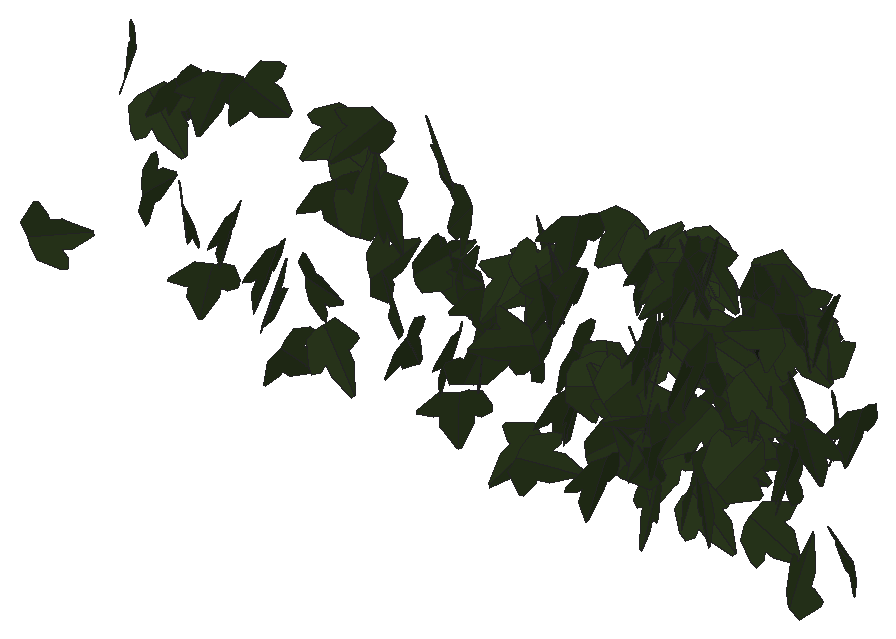
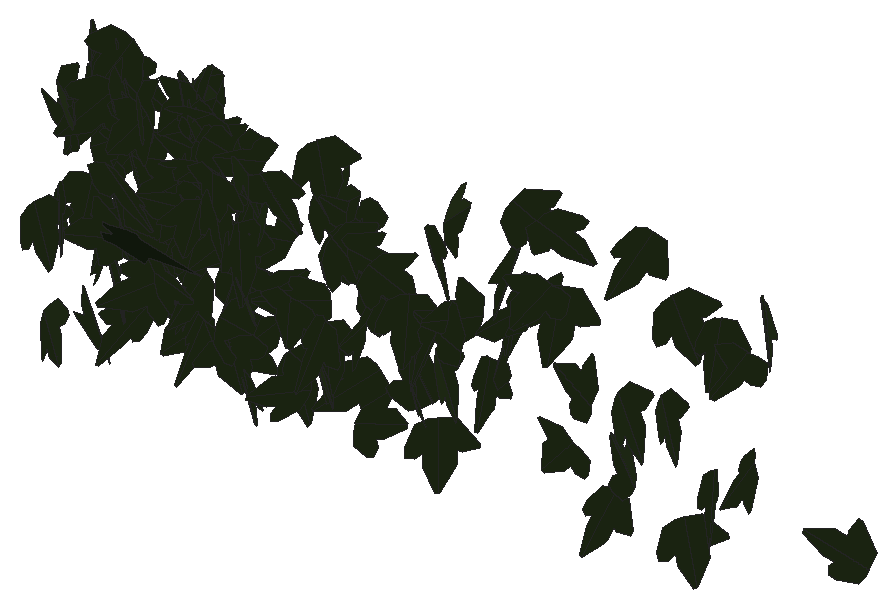
# SketchUp Ruby script. Lengths in inches.
U = 1.inch
M = Sketchup.active_model
def pt(a) = Geom::Point3d.new(a.map { |v| v * U })
def face(e, loops, mat)
  f = e.add_face(loops[0].map { |a| pt(a) })
  loops[1..].each { |l| e.add_face(l.map { |a| pt(a) }).erase! }
  f.material = f.back_material = mat if mat
  f
end
# faces: each face lists its corners as indices into pts; further lists are holes
def faces(e, pts, list, mat = nil) = list.each { |f| face(e, (f[0].is_a?(Array) ? f : [f]).map { |l| l.map { |i| pts[i] } }, mat) }
# xy, xz, yz: faces in a plane at the given z, y or x. An outline is a flat list of corners, or four numbers for a rectangle; further outlines are holes
def ring(l) = l.size == 4 ? [[l[0], l[1]], [l[2], l[1]], [l[2], l[3]], [l[0], l[3]]] : l.each_slice(2).to_a
def flat(e, list, mat, &to3) = list.each { |f| face(e, (f[0].is_a?(Array) ? f : [f]).map { |l| ring(l).map { |u, v| to3.(u, v) } }, mat) }
def xy(e, z, list, mat = nil) = flat(e, list, mat) { |x, y| [x, y, z] }
def xz(e, y, list, mat = nil) = flat(e, list, mat) { |x, z| [x, y, z] }
def yz(e, x, list, mat = nil) = flat(e, list, mat) { |y, z| [x, y, z] }
def lines(e, pts, list) = list.each { |a, b| e.add_line(pt(pts[a]), pt(pts[b])) }
# prism: a flat outline (further loops are holes) pulled along v
def prism(e, loops, v, mat = nil)
  f = face(e, loops, mat); d = Geom::Vector3d.new(v.map { |x| x * U })
  f.pushpull(f.normal.samedirection?(d) ? d.length : -d.length)
end
def box(e, o, s, mat = nil) = prism(e, [[o, [o[0] + s[0], o[1], o[2]], [o[0] + s[0], o[1] + s[1], o[2]], [o[0], o[1] + s[1], o[2]]]], [0, 0, s[2]], mat)
def at(x, y, z, deg = 0) = Geom::Transformation.translation(pt([x, y, z])) * Geom::Transformation.rotation(ORIGIN, Z_AXIS, deg.degrees)
def axes(o, x, y, z) = Geom::Transformation.new([*x, 0, *y, 0, *z, 0, *pt(o).to_a, 1])
def part(name) = M.definitions.add(name)
# library, detail: a bought-in or finely detailed component or shape, given as its bounding box
def library(name, o, s) = part(name).tap { |d| box(d.entities, o, s) }
def detail(e, o, s) = box(e.add_group.entities, o, s)
def put(e, d, t, mat = nil) = e.add_instance(d, t).tap { |i| i.material = mat if mat }
def group(e, t, mat = nil) = e.add_group.tap { |g| g.transformation = t; g.material = mat if mat }.entities
root = M.entities
M.materials.add("efeu1").color = [18, 25, 13]
M.materials.add("efeu2").color = [43, 57, 29]
c1 = part("ivyleaf_10")
p = [[0,0.5,-0.03],[-0.0625,2.02,-0.43],[-0.19,2.01,-0.46],[-0.54,1.05,-0.29],[-0.52,0.625,-0.18],[-0.83,0.76,-0.28],
  [-1.16,0.64,-0.33],[-1.15,0.33,-0.24],[-0.77,-0.39,0.02],[-0.3,-0.51,0.16],[0.04,-0.48,0.23],[-0.02,2.01,-0.4375],
  [-0.06,2.01,-0.43],[0.04,-0.49,0.23],[0.67,-0.49,0.14],[1.38,0.36,-0.2],[1.375,0.51,-0.24],[0.81,0.65,-0.19],
  [0.62,0.59,-0.15],[0.6,1.09,-0.28],[0.5,1.23,-0.31]]
faces(c1.entities,p,[[0,1,2,3,4,5,6,7,8,9,10],[11,12,0,13,14,15,16,17,18,19,20]],"efeu2")
c2 = part("ivyleaf_9")
p = [[1.54,2.16,1.25],[1.36,2.04,1.19],[-0.21,0.99,0.68],[-0.71,1.11,0.82],[-0.85,0.86,0.67],[-0.8,0.17,0.21],
  [-0.9,-0.01,0.1],[-0.67,-0.16,-0.02],[-0.08,-0.08,-0.05],[-0.03,-0.6,-0.4],[0.65,-0.88,-0.66],[0.83,-0.6,-0.49],
  [1.29,-0.42,-0.43],[1.8125,-0.07,-0.26],[1.21,0.44,0.15]]
faces(c2.entities,p,[[0,1,2,3,4,5,6,7,8,9,10,11,12,13,14]],"efeu1")
put(root,c1,axes([501.58,137.47,159.57],[-0.15363,-0.08574,0.63617],[0.63827,-0.09001,0.14201],[0.0683,0.64823,0.10386]))
put(root,c1,axes([514.61,137.29,163.09],[0.28468,-0.08203,-0.61214],[-0.58872,0.1677,-0.29626],[0.18669,0.65393,-0.00081]))
put(root,c1,axes([507.5,137.51,160.09],[-0.19823,-0.08508,0.65447],[-0.59816,-0.2656,-0.2157],[0.27888,-0.63015,0.00255]))
put(root,c1,axes([500.39,137.57,159.78],[0.13119,-0.67833,0.12845],[0.01858,-0.12724,-0.69088],[0.69014,0.13238,-0.00582]))
put(root,c1,axes([510.52,136.97,160.17],[0.20261,0.20728,-0.57368],[0.31352,0.48315,0.2853],[0.52324,-0.36976,0.0512]))
put(root,c1,axes([508.06,137.08,157.59],[-0.19672,-0.24079,-0.58709],[0.44123,0.38984,-0.30773],[0.45604,-0.48104,0.04448]))
put(root,c1,axes([508.8,137.75,162.04],[0.07103,-0.52918,0.35272],[0.1021,-0.34082,-0.53189],[0.62771,0.11532,0.04661]))
put(root,c1,axes([512.47,137.85,161.54],[0.1709,-0.54536,0.41093],[0.14339,-0.3855,-0.57124],[0.66762,0.22239,0.0175]))
put(root,c1,axes([512.6,137.52,158.25],[-0.20094,0.57916,-0.17977],[0.05958,-0.16961,-0.61302],[-0.60348,-0.20958,-0.00067]))
put(root,c1,axes([512.37,137.76,159.86],[0.27339,0.33514,-0.47041],[-0.33166,-0.335,-0.43142],[-0.47287,0.42872,0.03062]))
put(root,c1,axes([503.98,137.48,159.51],[-0.43148,0.46856,-0.05166],[-0.04085,0.0326,0.63691],[0.46963,0.43333,0.00794]))
put(root,c1,axes([514.19,137.28,161.55],[0.34109,0.43905,0.38721],[0.24422,0.30056,-0.55593],[-0.53203,0.41945,-0.00695]))
put(root,c1,axes([515.24,137.71,162.75],[-0.52008,0.25845,0.41449],[0.36412,-0.19845,0.58062],[0.3256,0.63475,0.01276]))
put(root,c1,axes([509.6,137.68,157.63],[-0.04447,-0.69393,0.08531],[-0.01168,-0.08473,-0.69533],[0.69906,-0.04556,-0.00619]))
put(root,c1,axes([493.99,137.42,158.09],[-0.22681,-0.0979,0.62095],[0.56047,0.26745,0.24689],[-0.28467,0.60456,-0.00867]))
put(root,c1,axes([503.05,137.83,163.91],[-0.27062,-0.33223,0.47396],[-0.26732,-0.39232,-0.42764],[0.51338,-0.37942,0.02716]))
put(root,c1,axes([501.97,137.59,158.23],[0.47834,0.05986,0.45963],[0.45841,0.03668,-0.48184],[-0.06862,0.66236,-0.01486]))
put(root,c1,axes([510.58,137.83,160.58],[-0.25371,0.07092,0.58722],[0.51638,-0.28506,0.25752],[0.28847,0.57266,0.05547]))
put(root,c1,axes([512.22,137.13,160.54],[0.14618,-0.30767,0.66519],[-0.30082,0.59334,0.34054],[-0.66832,-0.33436,-0.00778]))
put(root,c1,axes([512.1,137.95,163.47],[0.14526,-0.54386,0.4039],[0.09661,-0.39222,-0.56288],[0.67051,0.17433,-0.0064]))
put(root,c1,axes([511.49,137.15,159.2],[0.09626,-0.2164,-0.62084],[-0.05272,0.6229,-0.22529],[0.65536,0.08189,0.07306]))
put(root,c1,axes([504.39,137.35,159.15],[-0.02053,-0.52228,-0.39569],[-0.00995,0.39609,-0.52228],[0.65517,-0.01035,-0.02033]))
put(root,c1,axes([502.37,137.75,163.71],[0.45047,0.13049,-0.44841],[-0.42871,-0.13156,-0.46896],[-0.18522,0.62184,-0.00512]))
put(root,c1,axes([507.23,138.1,157.17],[-0.10202,-0.20529,0.60027],[0.06517,-0.60816,-0.19692],[0.63105,0.02961,0.11737]))
put(root,c1,axes([499.125,137.71,160.21],[0.15133,-0.61984,-0.00619],[-0.00174,0.00594,-0.63804],[0.61986,0.15134,-0.00028]))
put(root,c1,axes([513.92,137.83,161.26],[0.58198,-0.29155,0.13847],[0.1229,-0.06383,-0.65092],[0.29845,0.59481,-0.00198]))
put(root,c1,axes([511.1,137.97,159.48],[-0.12286,-0.13664,0.64471],[-0.47353,-0.43782,-0.18303],[0.45835,-0.48894,-0.01628]))
put(root,c1,axes([503.74,137.16,160.81],[0.06513,0.02379,-0.69063],[0.16084,0.67412,0.03839],[0.67206,-0.16364,0.05774]))
put(root,c1,axes([508.13,137.52,161.73],[-0.54225,0.28859,0.2173],[-0.19538,0.09539,-0.61422],[-0.30386,-0.57633,0.00715]))
put(root,c1,axes([505.3,137.86,159.23],[0.23403,-0.6359,0.06055],[0.02155,-0.05659,-0.67759],[0.63841,0.23502,0.00068]))
put(root,c1,axes([512.16,137.46,163.83],[0.09475,-0.49313,-0.41549],[0.07959,0.42569,-0.48708],[0.6399,0.02008,0.1221]))
put(root,c1,axes([503.62,137.49,162.4],[-0.23965,0.67302,0.18709],[-0.06207,0.17649,-0.71442],[-0.69578,-0.24755,-0.0007]))
put(root,c1,axes([515.09,137.59,163.5],[-0.26481,0.0617,0.60507],[-0.59807,0.09356,-0.27128],[-0.11057,-0.65382,0.01827]))
put(root,c1,axes([510.15,137.78,159.35],[0.38141,0.22713,0.37776],[-0.35725,-0.15456,0.43499],[0.294,-0.48247,0.03849]))
put(root,c1,axes([514.22,138,163.42],[0.08021,-0.60947,0.22363],[0.02613,-0.22211,-0.61472],[0.64868,0.08431,-0.00289]))
put(root,c1,axes([499.92,137.48,163.98],[-0.20069,-0.48468,-0.46335],[0.28157,0.37804,-0.51739],[0.60855,-0.33475,0.08659]))
put(root,c1,axes([512.58,137.48,163.08],[-0.2335,0.33408,-0.55742],[-0.40881,0.38491,0.40194],[0.50517,0.46592,0.06763]))
put(root,c1,axes([513.02,137.53,159.33],[-0.41953,-0.26297,-0.51972],[0.44447,0.26942,-0.4951],[0.37644,-0.61117,0.00537]))
put(root,c1,axes([512.75,137.66,161.43],[-0.3029,0.07771,0.61393],[-0.61329,0.05355,-0.30936],[-0.08261,-0.68249,0.04563]))
put(root,c1,axes([512.39,137.73,162.93],[0.33621,-0.5789,0.1251],[-0.05948,0.11013,0.66944],[-0.58927,-0.34141,0.00381]))
put(root,c1,axes([515.05,137.77,156.35],[0.63278,-0.35767,-0.06101],[0.06182,-0.01458,0.72666],[-0.35753,-0.63555,0.01767]))
put(root,c1,axes([510.98,137.43,161.3125],[0.02898,-0.34464,-0.53511],[0.00418,0.53575,-0.34482],[0.63647,0.01217,0.02664]))
put(root,c1,axes([512.32,137.69,157.68],[0.41857,0.19512,0.47103],[0.42864,0.19531,-0.46181],[-0.27606,0.59911,-0.00286]))
put(root,c1,axes([512,137.78,162.14],[0.1016,-0.05206,-0.67101],[0.67038,-0.0523,0.10556],[-0.05963,-0.67664,0.04347]))
put(root,c1,axes([508.74,137.9,163.35],[-0.28874,-0.58596,0.0746],[-0.0238,-0.07142,-0.65316],[0.59021,-0.28954,0.01015]))
put(root,c1,axes([513.41,137.32,158.94],[0.29263,0.2796,-0.64011],[0.32859,0.55732,0.39366],[0.61639,-0.42984,0.09404]))
put(root,c1,axes([515.16,137.61,161.26],[-0.28218,0.20796,-0.5476],[-0.42805,0.34171,0.35035],[0.39985,0.51257,-0.01139]))
put(root,c1,axes([496.41,137.6,163.58],[0.20439,-0.41925,-0.46224],[-0.21425,0.4097,-0.46633],[0.58612,0.29596,-0.00927]))
put(root,c1,axes([508,138.13,161.43],[-0.13132,-0.53477,0.34231],[-0.07178,-0.33481,-0.55059],[0.63088,-0.14941,0.00861]))
put(root,c1,axes([500.18,137.77,158.18],[0.26893,-0.56118,0.14321],[-0.05915,0.13045,0.62229],[-0.57614,-0.27534,0.00296]))
put(root,c1,axes([511.55,138.28,162.74],[-0.1057,-0.3157,0.54538],[-0.17721,-0.51579,-0.33292],[0.60473,-0.20633,-0.00223]))
put(root,c1,axes([507.64,137.64,161.86],[0.32023,0.18257,-0.50394],[0.45623,0.23763,0.36195],[0.32341,-0.51599,-0.01162]))
put(root,c1,axes([510.76,137.92,157.84],[-0.45919,0.08336,-0.43854],[-0.43543,0.05495,0.46637],[0.09833,0.63258,0.01728]))
put(root,c1,axes([508.375,137.64,162.11],[-0.29467,0.27244,-0.56884],[-0.40751,0.39697,0.40122],[0.48139,0.50281,-0.00855]))
put(root,c1,axes([514.34,137.86,164.02],[-0.62669,0.08538,-0.31229],[0.30815,-0.05139,-0.63242],[-0.0993,-0.6983,0.00836]))
put(root,c1,axes([502.03,137.84,161.96],[-0.40152,-0.56364,-0.16539],[0.09741,0.13367,-0.69203],[0.57928,-0.41316,0.00174]))
put(root,c1,axes([506.74,138.31,161.24],[-0.27553,-0.35239,0.45368],[-0.06106,-0.48235,-0.41173],[0.5712,-0.22154,0.17483]))
put(root,c1,axes([507.54,138.33,161.53],[-0.33305,-0.14414,0.53416],[-0.24565,-0.52013,-0.29351],[0.49574,-0.35456,0.21342]))
put(root,c1,axes([510.68,138.1,157.19],[0.52907,-0.37381,0.08968],[0.07712,-0.04624,-0.64777],[0.3766,0.53462,0.00667]))
put(root,c1,axes([496.9,137.83,162.3],[0.44671,0.33533,0.35778],[0.28944,0.21036,-0.55854],[-0.39582,0.53226,-0.00466]))
put(root,c1,axes([498.43,138.18,163.18],[-0.2959,-0.56367,0.2269],[-0.07465,-0.21674,-0.63577],[0.60302,-0.30342,0.03264]))
put(root,c1,axes([508.4,137.98,158.875],[-0.06951,-0.67732,-0.12922],[0.01807,0.12804,-0.68086],[0.6893,-0.07166,0.00482]))
put(root,c1,axes([509,137.76,159.51],[0.01037,-0.08525,-0.65903],[0.61204,0.25796,-0.02374],[0.25884,-0.60654,0.08254]))
put(root,c1,axes([505.72,137.98,158.54],[-0.21318,-0.60311,0.18181],[0.06742,0.169,0.63963],[-0.6263,0.22347,0.00697]))
put(root,c1,axes([515.24,137.96,160.25],[-0.63723,-0.02421,-0.01622],[0.01623,-0.00002,-0.63769],[0.0242,-0.63743,0.00063]))
put(root,c1,axes([502.79,137.69,161.51],[0.11907,0.60555,-0.37945],[0.05504,0.37577,0.61695],[0.71249,-0.13023,0.01576]))
put(root,c1,axes([505.27,138.07,157.625],[-0.46195,-0.46919,0.00578],[-0.00095,-0.00717,-0.65843],[0.46923,-0.46193,0.00436]))
put(root,c1,axes([511.28,138.42,162.95],[-0.23339,-0.252,0.47785],[-0.16783,-0.44383,-0.32918],[0.54051,-0.24663,0.10412]))
put(root,c1,axes([510.68,138.57,158.71],[-0.08099,-0.43169,0.57146],[0.08095,-0.57694,-0.42436],[0.7116,0.0165,0.11332]))
put(root,c1,axes([500.61,137.82,157.37],[-0.17442,-0.43726,-0.4379],[0.14775,0.41238,-0.47062],[0.60093,-0.2283,-0.01139]))
put(root,c1,axes([510.98,137.91,161.64],[0.23686,-0.49707,-0.37628],[-0.06098,0.38212,-0.54317],[0.62044,0.22732,0.09027]))
put(root,c1,axes([497.39,137.98,162.88],[-0.16384,-0.56641,-0.24556],[0.05753,0.23895,-0.58954],[0.61467,-0.17334,-0.01028]))
put(root,c1,axes([507.62,138.54,161.67],[-0.10119,-0.56434,0.41807],[0.04521,-0.42674,-0.56511],[0.70087,-0.05395,0.09681]))
put(root,c1,axes([506.05,138.16,160.51],[-0.39088,-0.51791,-0.06961],[0.03677,0.05945,-0.64883],[0.52128,-0.39255,-0.00643]))
put(root,c1,axes([511,138.57,161.52],[-0.05085,0.05309,0.64855],[0.48285,-0.43302,0.07331],[0.43622,0.48549,-0.00554]))
put(root,c1,axes([512.08,138.16,163.57],[0.4761,0.09577,0.47932],[0.45196,0.16854,-0.48261],[-0.18613,0.65422,0.05416]))
put(root,c1,axes([511.53,138.49,163.59],[-0.47031,-0.32277,-0.33963],[0.4934,-0.34963,-0.27419],[-0.04963,-0.41719,0.49256]))
put(root,c1,axes([510.46,138.4,162.97],[0.14899,-0.71611,0.08053],[0.02229,-0.07761,-0.73142],[0.72028,0.15053,0.00598]))
put(root,c1,axes([512.02,137.95,157.85],[0.09296,-0.48285,-0.47024],[0.11276,0.47915,-0.4697],[0.6645,-0.01375,0.14549]))
put(root,c1,axes([513.23,138.52,163.33],[0.22331,-0.52002,0.29566],[0.2141,-0.2252,-0.5578],[0.55856,0.29422,0.0956]))
put(root,c1,axes([510.38,138.59,159.87],[0.43984,-0.42576,0.38493],[0.26133,-0.28322,-0.61188],[0.51102,0.51129,-0.0184]))
put(root,c1,axes([505.38,138.12,162.45],[0.36404,-0.33146,-0.44071],[-0.29429,0.32981,-0.49115],[0.46635,0.46687,0.03408]))
put(root,c1,axes([513.29,138.05,159.77],[-0.19356,-0.16323,0.66632],[0.51912,0.41776,0.25314],[-0.44849,0.554,0.00543]))
put(root,c1,axes([514.8,137.98,162.57],[0.21447,0.53764,0.39935],[0.1443,0.37239,-0.57883],[-0.654,0.25848,0.00325]))
put(root,c1,axes([508.31,138.42,158.76],[0.32641,-0.58292,0.02596],[0.01559,-0.02102,-0.66808],[0.58329,0.32677,0.00334]))
put(root,c1,axes([513.86,137.99,157.52],[0.1009,0.49755,0.43375],[0.10087,0.42201,-0.50755],[-0.65232,0.14221,-0.01139]))
put(root,c1,axes([504.53,137.91,160.77],[0.03308,-0.17729,0.62435],[0.01747,0.62518,0.1766],[-0.6488,0.00779,0.03659]))
put(root,c1,axes([504.82,138.14,163.21],[-0.23863,0.37215,-0.48251],[-0.34316,0.34613,0.43668],[0.50354,0.41225,0.06894]))
put(root,c1,axes([514.28,138.31,158.98],[0.36452,-0.5007,-0.32821],[-0.19926,0.26089,-0.6193],[0.56455,0.41537,-0.00666]))
put(root,c1,axes([512.53,138.13,161.45],[0.23168,0.27516,0.53506],[0.35545,0.40001,-0.35962],[-0.48545,0.42422,-0.00796]))
put(root,c1,axes([514.75,137.96,159.07],[0.02282,-0.05324,0.7025],[-0.45063,0.53918,0.0555],[-0.54154,-0.45091,-0.01658]))
put(root,c1,axes([515.2,138.79,163.13],[0.29976,-0.49721,0.28868],[0.1271,-0.2602,-0.58014],[0.56072,0.3248,-0.02283]))
put(root,c1,axes([510.67,138.58,158.1],[0.46285,0.45478,-0.11108],[-0.08115,-0.0759,-0.64888],[-0.46106,0.46991,0.0027]))
put(root,c1,axes([507.39,138.04,159.53],[0.06725,0.10616,-0.63271],[-0.02956,0.63602,0.10358],[0.64088,0.01819,0.07117]))
put(root,c1,axes([504.43,138.59,160.4375],[-0.13772,-0.01356,0.62307],[0.62271,0.02253,0.13814],[-0.02492,0.63771,0.00837]))
put(root,c1,axes([505.34,138.82,159.08],[0.38392,-0.33991,0.40081],[0.32024,-0.24226,-0.51219],[0.41669,0.49935,0.02435]))
put(root,c1,axes([497.82,138.63,158],[-0.40892,-0.47441,0.11149],[-0.06554,-0.09068,-0.62625],[0.4829,-0.41403,0.00942]))
put(root,c1,axes([510.43,138.56,160.91],[-0.01994,-0.71606,-0.12535],[0.01536,0.12496,-0.71624],[0.72679,-0.02229,0.0117]))
put(root,c1,axes([512.2,138.21,160.91],[0.17854,0.16685,-0.59298],[0.44333,0.39384,0.2443],[0.42769,-0.4779,-0.0057]))
put(root,c1,axes([508.92,138.64,159.8],[0.61941,0.02777,0.17996],[0.17908,0.0226,-0.61988],[-0.03296,0.64463,0.01398]))
put(root,c1,axes([514.4,138.4,163.06],[-0.39796,-0.23527,-0.49108],[0.43236,0.23322,-0.46211],[0.33101,-0.58748,0.01321]))
put(root,c1,axes([515.46,138.51,161.97],[0.53933,-0.14786,0.33847],[-0.32726,0.08644,0.55923],[-0.17125,-0.63085,-0.00271]))
put(root,c1,axes([511.46,138.87,162.5],[-0.47856,-0.30155,-0.25948],[0.42238,-0.32664,-0.3118],[0.01627,-0.38975,0.46206]))
put(root,c1,axes([514.17,138.29,160.85],[0.13118,-0.12149,-0.63926],[-0.34864,0.53749,-0.17369],[0.54942,0.37008,0.04241]))
put(root,c1,axes([510.28,138.18,162.77],[0.24257,0.21093,-0.58955],[0.24809,0.54812,0.29818],[0.5749,-0.32553,0.12007]))
put(root,c1,axes([496.4,138.1875,159.8125],[0.03613,-0.15139,-0.63183],[0.03534,0.63232,-0.14948],[0.64875,-0.02602,0.04333]))
put(root,c1,axes([513.29,138.67,162.9375],[-0.51304,0.19167,-0.37538],[0.34673,-0.14427,-0.54755],[-0.23963,-0.61911,0.01138]))
put(root,c1,axes([510.79,138.42,160.81],[0.31212,0.32673,0.47763],[0.32445,0.35055,-0.45183],[-0.47918,0.45018,0.00518]))
put(root,c1,axes([501.86,138.58,162.61],[0.41885,0.30393,0.38857],[0.3032,0.24349,-0.51728],[-0.38914,0.51685,0.0152]))
put(root,c1,axes([511.77,138.3125,159.26],[-0.03042,-0.29378,-0.60787],[0.08589,0.60186,-0.29517],[0.66965,-0.09054,0.01024]))
put(root,c1,axes([512.84,138.54,158.99],[-0.25662,-0.15825,-0.61335],[0.55124,0.27023,-0.30036],[0.31206,-0.60748,0.02617]))
put(root,c1,axes([497.16,138.58,159.39],[-0.45427,0.31996,0.33371],[-0.29149,0.16492,-0.55492],[-0.35885,-0.53901,0.02831]))
put(root,c1,axes([513.97,138.77,159.84],[0.13085,-0.04769,0.62357],[0.6002,0.18856,-0.11153],[-0.1757,0.60861,0.08342]))
put(root,c1,axes([509.01,138.4,157.55],[-0.02684,-0.13598,0.63034],[0.05176,0.6284,0.13776],[-0.64276,0.05628,-0.01523]))
put(root,c1,axes([505.09,138.51,160.35],[-0.17881,0.34148,0.51919],[-0.24526,0.45762,-0.38545],[-0.57098,-0.3035,0.00297]))
put(root,c1,axes([515.72,138.67,157.04],[0.27487,-0.00481,-0.58183],[-0.35408,0.50924,-0.17148],[0.46171,0.39339,0.21487]))
put(root,c1,axes([509.22,139.0625,162.96],[0.56022,0.0038,-0.30246],[-0.30227,0.03091,-0.55948],[0.01135,0.6359,0.029]))
put(root,c1,axes([515.31,138.78,160.31],[0.23514,-0.34657,-0.49904],[-0.18969,0.46648,-0.41334],[0.5772,0.29449,0.06746]))
put(root,c1,axes([510.65,139.16,162.07],[-0.00156,-0.66588,-0.03591],[0.00081,0.03591,-0.66588],[0.66685,-0.00161,0.00072]))
put(root,c1,axes([512.32,139.04,159.46],[0.10679,0.103,0.62596],[-0.63185,0.07391,0.09563],[-0.0566,-0.63069,0.11343]))
put(root,c1,axes([507.93,138.84,159.51],[-0.02251,-0.46202,-0.52873],[0.06087,0.52573,-0.46198],[0.69951,-0.06062,0.02318]))
put(root,c1,axes([515.42,139.45,160.15],[-0.08351,-0.62761,0.08149],[-0.00459,-0.08159,-0.63311],[0.63286,-0.08341,0.00616]))
put(root,c1,axes([510.46,139.42,162.75],[0.62705,-0.04298,0.16909],[0.16898,-0.00736,-0.62851],[0.04341,0.64941,0.00407]))
put(root,c1,axes([511.03,139.34,161.82],[0.24183,0.59832,0.10775],[0.03936,0.10031,-0.64535],[-0.60667,0.24502,0.00108]))
put(root,c2,axes([512.56,140.25,161.01],[-0.69017,0.20052,-0.00265],[-0.0983,-0.29761,-0.6168],[-0.19298,-0.56553,0.32365]))
put(root,c1,axes([512.74,140.23,162.38],[-0.74922,0.28567,0.20476],[-0.36137,-0.4345,-0.57046],[-0.09907,-0.57552,0.53231]))
